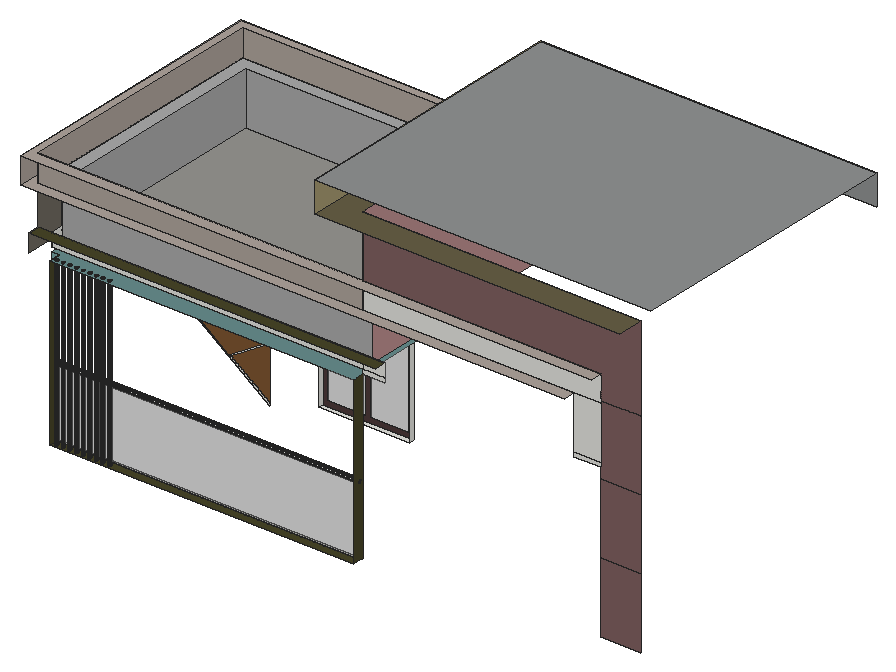
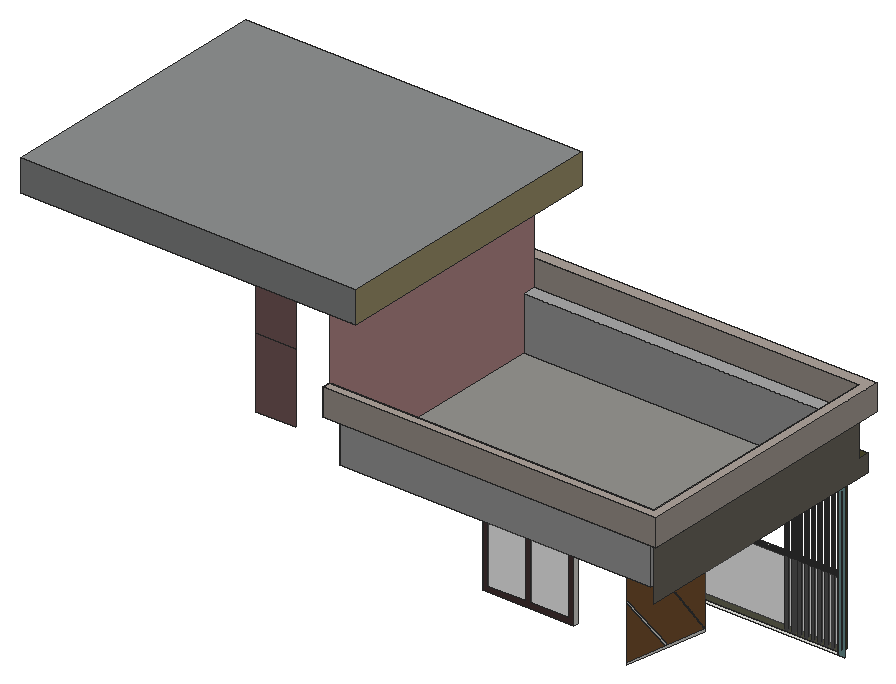
# SketchUp Ruby script. Lengths in inches.
U = 1.inch
M = Sketchup.active_model
def pt(a) = Geom::Point3d.new(a.map { |v| v * U })
def face(e, loops, mat)
  f = e.add_face(loops[0].map { |a| pt(a) })
  loops[1..].each { |l| e.add_face(l.map { |a| pt(a) }).erase! }
  f.material = f.back_material = mat if mat
  f
end
# faces: each face lists its corners as indices into pts; further lists are holes
def faces(e, pts, list, mat = nil) = list.each { |f| face(e, (f[0].is_a?(Array) ? f : [f]).map { |l| l.map { |i| pts[i] } }, mat) }
# xy, xz, yz: faces in a plane at the given z, y or x. An outline is a flat list of corners, or four numbers for a rectangle; further outlines are holes
def ring(l) = l.size == 4 ? [[l[0], l[1]], [l[2], l[1]], [l[2], l[3]], [l[0], l[3]]] : l.each_slice(2).to_a
def flat(e, list, mat, &to3) = list.each { |f| face(e, (f[0].is_a?(Array) ? f : [f]).map { |l| ring(l).map { |u, v| to3.(u, v) } }, mat) }
def xy(e, z, list, mat = nil) = flat(e, list, mat) { |x, y| [x, y, z] }
def xz(e, y, list, mat = nil) = flat(e, list, mat) { |x, z| [x, y, z] }
def yz(e, x, list, mat = nil) = flat(e, list, mat) { |y, z| [x, y, z] }
def lines(e, pts, list) = list.each { |a, b| e.add_line(pt(pts[a]), pt(pts[b])) }
# prism: a flat outline (further loops are holes) pulled along v
def prism(e, loops, v, mat = nil)
  f = face(e, loops, mat); d = Geom::Vector3d.new(v.map { |x| x * U })
  f.pushpull(f.normal.samedirection?(d) ? d.length : -d.length)
end
def box(e, o, s, mat = nil) = prism(e, [[o, [o[0] + s[0], o[1], o[2]], [o[0] + s[0], o[1] + s[1], o[2]], [o[0], o[1] + s[1], o[2]]]], [0, 0, s[2]], mat)
def at(x, y, z, deg = 0) = Geom::Transformation.translation(pt([x, y, z])) * Geom::Transformation.rotation(ORIGIN, Z_AXIS, deg.degrees)
def axes(o, x, y, z) = Geom::Transformation.new([*x, 0, *y, 0, *z, 0, *pt(o).to_a, 1])
def part(name) = M.definitions.add(name)
# library, detail: a bought-in or finely detailed component or shape, given as its bounding box
def library(name, o, s) = part(name).tap { |d| box(d.entities, o, s) }
def detail(e, o, s) = box(e.add_group.entities, o, s)
def put(e, d, t, mat = nil) = e.add_instance(d, t).tap { |i| i.material = mat if mat }
def group(e, t, mat = nil) = e.add_group.tap { |g| g.transformation = t; g.material = mat if mat }.entities
root = M.entities
M.materials.add("[0057_DarkKhaki]").color = [71, 69, 40]
M.materials.add("[0089_PaleTurquoise]").color = [103, 140, 140]
M.materials.add("[0089_PaleTurquoise]1").color = [120, 163, 163]
M.materials.add("[0119_RosyBrown]").color = [127, 96, 96]
M.materials.add("[0119_RosyBrown]1").color = [76, 58, 58]
M.materials.add("[0119_RosyBrown]2").color = [188, 143, 143]
M.materials.add("[0132_LightGray]1").color = [169, 169, 169]
M.materials.add("[Blacktop Old 02]").color = [143, 145, 145]
M.materials.add("[Cladding Stucco White]").color = [173, 163, 155]
M.materials.add("[Cladding Weathered]").color = [111, 105, 96]
M.materials.add("[Granite Light Gray]1").color = [149, 148, 144]
M.materials.add("[Translucent Glass Gray]").color = [130, 130, 130]
M.materials["[Translucent Glass Gray]"].alpha = 0.5
M.materials.add("[Translucent Glass Gray]1").color = [128, 128, 128]
M.materials["[Translucent Glass Gray]1"].alpha = 0.5
M.materials.add("[Wood Floor]").color = [124, 84, 49]
M.materials.add("[Wood Lumber ButtJoined]").color = [102, 94, 69]
M.materials.add("[Wood Lumber ButtJoined]3").color = [164, 152, 112]
xy(root,2010,[[306.11,174.36,305.08,174.5,304.11,174.9,303.29,175.53,302.65,176.36,302.25,177.32,302.11,178.36,302.25,179.4,302.65,180.36,303.29,181.1875,304.11,181.82,305.08,182.22,306.11,182.36,307.15,182.22,308.11,181.82,308.94,181.1875,309.58,180.36,309.98,179.4,310.11,178.36,309.98,177.32,309.58,176.36,308.94,175.53,308.11,174.9,307.15,174.5],[296.4,189.72,1122,198]])
xy(root,2010,[[[296.4,167,1122,189.72],[324.11,174.36,323.08,174.5,322.11,174.9,321.29,175.53,320.65,176.36,320.25,177.32,320.11,178.36,320.25,179.4,320.65,180.36,321.29,181.1875,322.11,181.82,323.08,182.22,324.11,182.36,325.15,182.22,326.11,181.82,326.94,181.1875,327.58,180.36,327.98,179.4,328.11,178.36,327.98,177.32,327.58,176.36,326.94,175.53,326.11,174.9,325.15,174.5],[342.11,174.36,341.08,174.5,340.11,174.9,339.29,175.53,338.65,176.36,338.25,177.32,338.11,178.36,338.25,179.4,338.65,180.36,339.29,181.1875,340.11,181.82,341.08,182.22,342.11,182.36,343.15,182.22,344.11,181.82,344.94,181.1875,345.58,180.36,345.98,179.4,346.11,178.36,345.98,177.32,345.58,176.36,344.94,175.53,344.11,174.9,343.15,174.5],[360.11,174.36,359.08,174.5,358.11,174.9,357.29,175.53,356.65,176.36,356.25,177.32,356.11,178.36,356.25,179.4,356.65,180.36,357.29,181.1875,358.11,181.82,359.08,182.22,360.11,182.36,361.15,182.22,362.11,181.82,362.94,181.1875,363.58,180.36,363.98,179.4,364.11,178.36,363.98,177.32,363.58,176.36,362.94,175.53,362.11,174.9,361.15,174.5],[378.11,174.36,377.08,174.5,376.11,174.9,375.29,175.53,374.65,176.36,374.25,177.32,374.11,178.36,374.25,179.4,374.65,180.36,375.29,181.1875,376.11,181.82,377.08,182.22,378.11,182.36,379.15,182.22,380.11,181.82,380.94,181.1875,381.58,180.36,381.98,179.4,382.11,178.36,381.98,177.32,381.58,176.36,380.94,175.53,380.11,174.9,379.15,174.5],[396.11,174.36,395.08,174.5,394.11,174.9,393.29,175.53,392.65,176.36,392.25,177.32,392.11,178.36,392.25,179.4,392.65,180.36,393.29,181.1875,394.11,181.82,395.08,182.22,396.11,182.36,397.15,182.22,398.11,181.82,398.94,181.1875,399.58,180.36,399.98,179.4,400.11,178.36,399.98,177.32,399.58,176.36,398.94,175.53,398.11,174.9,397.15,174.5],[414.11,174.36,413.08,174.5,412.11,174.9,411.29,175.53,410.65,176.36,410.25,177.32,410.11,178.36,410.25,179.4,410.65,180.36,411.29,181.1875,412.11,181.82,413.08,182.22,414.11,182.36,415.15,182.22,416.11,181.82,416.94,181.1875,417.58,180.36,417.98,179.4,418.11,178.36,417.98,177.32,417.58,176.36,416.94,175.53,416.11,174.9,415.15,174.5],[432.11,174.36,431.08,174.5,430.11,174.9,429.29,175.53,428.65,176.36,428.25,177.32,428.11,178.36,428.25,179.4,428.65,180.36,429.29,181.1875,430.11,181.82,431.08,182.22,432.11,182.36,433.15,182.22,434.11,181.82,434.94,181.1875,435.58,180.36,435.98,179.4,436.11,178.36,435.98,177.32,435.58,176.36,434.94,175.53,434.11,174.9,433.15,174.5],[450.11,174.36,449.08,174.5,448.11,174.9,447.29,175.53,446.65,176.36,446.25,177.32,446.11,178.36,446.25,179.4,446.65,180.36,447.29,181.1875,448.11,181.82,449.08,182.22,450.11,182.36,451.15,182.22,452.11,181.82,452.94,181.1875,453.58,180.36,453.98,179.4,454.11,178.36,453.98,177.32,453.58,176.36,452.94,175.53,452.11,174.9,451.15,174.5],[306.11,174.36,305.08,174.5,304.11,174.9,303.29,175.53,302.65,176.36,302.25,177.32,302.11,178.36,302.25,179.4,302.65,180.36,303.29,181.1875,304.11,181.82,305.08,182.22,306.11,182.36,307.15,182.22,308.11,181.82,308.94,181.1875,309.58,180.36,309.98,179.4,310.11,178.36,309.98,177.32,309.58,176.36,308.94,175.53,308.11,174.9,307.15,174.5]]],"[0057_DarkKhaki]")
xy(root,2088,[[726,546,973.25,558]])
xy(root,2374.11,[[373.89,546,586.11,552]])
xy(root,2388,[[726,546,973.25,558]])
xy(root,2460,[[411.39,218.73,408.29,219.14,405.39,220.34,402.91,222.25,401,224.73,399.8,227.625,399.39,230.73,399.8,233.84,401,236.73,402.91,239.22,405.39,241.125,408.29,242.32,411.39,242.73,414.5,242.32,417.39,241.125,419.88,239.22,421.79,236.73,422.99,233.84,423.39,230.73,422.99,227.625,421.79,224.73,419.88,222.25,417.39,220.34,414.5,219.14],[735.39,218.73,732.29,219.14,729.39,220.34,726.91,222.25,725,224.73,723.8,227.625,723.39,230.73,723.8,233.84,725,236.73,726.91,239.22,729.39,241.125,732.29,242.32,735.39,242.73,738.5,242.32,741.39,241.125,743.88,239.22,745.79,236.73,746.99,233.84,747.39,230.73,746.99,227.625,745.79,224.73,743.88,222.25,741.39,220.34,738.5,219.14],[1059.39,218.73,1056.29,219.14,1053.39,220.34,1050.91,222.25,1049,224.73,1047.8,227.625,1047.39,230.73,1047.8,233.84,1049,236.73,1050.91,239.22,1053.39,241.125,1056.29,242.32,1059.39,242.73,1062.5,242.32,1065.39,241.125,1067.88,239.22,1069.79,236.73,1070.99,233.84,1071.39,230.73,1070.99,227.625,1069.79,224.73,1067.88,222.25,1065.39,220.34,1062.5,219.14],[411.39,338.73,408.29,339.14,405.39,340.34,402.91,342.25,401,344.73,399.8,347.625,399.39,350.73,399.8,353.84,401,356.73,402.91,359.22,405.39,361.125,408.29,362.32,411.39,362.73,414.5,362.32,417.39,361.125,419.88,359.22,421.79,356.73,422.99,353.84,423.39,350.73,422.99,347.625,421.79,344.73,419.88,342.25,417.39,340.34,414.5,339.14],[735.39,338.73,732.29,339.14,729.39,340.34,726.91,342.25,725,344.73,723.8,347.625,723.39,350.73,723.8,353.84,725,356.73,726.91,359.22,729.39,361.125,732.29,362.32,735.39,362.73,738.5,362.32,741.39,361.125,743.88,359.22,745.79,356.73,746.99,353.84,747.39,350.73,746.99,347.625,745.79,344.73,743.88,342.25,741.39,340.34,738.5,339.14],
  [1059.39,338.73,1056.29,339.14,1053.39,340.34,1050.91,342.25,1049,344.73,1047.8,347.625,1047.39,350.73,1047.8,353.84,1049,356.73,1050.91,359.22,1053.39,361.125,1056.29,362.32,1059.39,362.73,1062.5,362.32,1065.39,361.125,1067.88,359.22,1069.79,356.73,1070.99,353.84,1071.39,350.73,1070.99,347.625,1069.79,344.73,1067.88,342.25,1065.39,340.34,1062.5,339.14]])
xy(root,2460,[[[296.4,167,296.4,198,276,198,276,546,1122,546,1122,167],[1059.39,218.73,1062.5,219.14,1065.39,220.34,1067.88,222.25,1069.79,224.73,1070.99,227.625,1071.39,230.73,1070.99,233.84,1069.79,236.73,1067.88,239.22,1065.39,241.125,1062.5,242.32,1059.39,242.73,1056.29,242.32,1053.39,241.125,1050.91,239.22,1049,236.73,1047.8,233.84,1047.39,230.73,1047.8,227.625,1049,224.73,1050.91,222.25,1053.39,220.34,1056.29,219.14],[411.39,218.73,414.5,219.14,417.39,220.34,419.88,222.25,421.79,224.73,422.99,227.625,423.39,230.73,422.99,233.84,421.79,236.73,419.88,239.22,417.39,241.125,414.5,242.32,411.39,242.73,408.29,242.32,405.39,241.125,402.91,239.22,401,236.73,399.8,233.84,399.39,230.73,399.8,227.625,401,224.73,402.91,222.25,405.39,220.34,408.29,219.14],[411.39,338.73,414.5,339.14,417.39,340.34,419.88,342.25,421.79,344.73,422.99,347.625,423.39,350.73,422.99,353.84,421.79,356.73,419.88,359.22,417.39,361.125,414.5,362.32,411.39,362.73,408.29,362.32,405.39,361.125,402.91,359.22,401,356.73,399.8,353.84,399.39,350.73,399.8,347.625,401,344.73,402.91,342.25,405.39,340.34,408.29,339.14],[735.39,338.73,738.5,339.14,741.39,340.34,743.88,342.25,745.79,344.73,746.99,347.625,747.39,350.73,746.99,353.84,745.79,356.73,743.88,359.22,741.39,361.125,738.5,362.32,735.39,362.73,732.29,362.32,729.39,361.125,726.91,359.22,725,356.73,723.8,353.84,723.39,350.73,723.8,347.625,725,344.73,726.91,342.25,729.39,340.34,732.29,339.14],[1059.39,338.73,1062.5,339.14,1065.39,340.34,1067.88,342.25,1069.79,344.73,1070.99,347.625,1071.39,350.73,1070.99,353.84,1069.79,356.73,1067.88,359.22,1065.39,361.125,1062.5,362.32,1059.39,362.73,1056.29,362.32,1053.39,361.125,1050.91,359.22,1049,356.73,1047.8,353.84,1047.39,350.73,1047.8,347.625,1049,344.73,1050.91,342.25,1053.39,340.34,1056.29,339.14],[735.39,218.73,738.5,219.14,741.39,220.34,743.88,222.25,745.79,224.73,746.99,227.625,747.39,230.73,746.99,233.84,745.79,236.73,743.88,239.22,741.39,241.125,738.5,242.32,735.39,242.73,732.29,242.32,729.39,241.125,726.91,239.22,725,236.73,723.8,233.84,723.39,230.73,723.8,227.625,725,224.73,726.91,222.25,729.39,220.34,732.29,219.14],[306.11,174.36,307.15,174.5,308.11,174.9,308.94,175.53,309.58,176.36,309.98,177.32,310.11,178.36,309.98,179.4,309.58,180.36,308.94,181.1875,308.11,181.82,307.15,182.22,306.11,182.36,305.08,182.22,304.11,181.82,303.29,181.1875,302.65,180.36,302.25,179.4,302.11,178.36,302.25,177.32,302.65,176.36,303.29,175.53,304.11,174.9,305.08,174.5],[324.11,174.36,325.15,174.5,326.11,174.9,326.94,175.53,327.58,176.36,327.98,177.32,328.11,178.36,327.98,179.4,327.58,180.36,326.94,181.1875,326.11,181.82,325.15,182.22,324.11,182.36,323.08,182.22,322.11,181.82,321.29,181.1875,320.65,180.36,320.25,179.4,320.11,178.36,320.25,177.32,320.65,176.36,321.29,175.53,322.11,174.9,323.08,174.5],[342.11,174.36,343.15,174.5,344.11,174.9,344.94,175.53,345.58,176.36,345.98,177.32,346.11,178.36,345.98,179.4,345.58,180.36,344.94,181.1875,344.11,181.82,343.15,182.22,342.11,182.36,341.08,182.22,340.11,181.82,339.29,181.1875,338.65,180.36,338.25,179.4,338.11,178.36,338.25,177.32,338.65,176.36,339.29,175.53,340.11,174.9,341.08,174.5],[360.11,174.36,361.15,174.5,362.11,174.9,362.94,175.53,363.58,176.36,363.98,177.32,364.11,178.36,363.98,179.4,363.58,180.36,362.94,181.1875,362.11,181.82,361.15,182.22,360.11,182.36,359.08,182.22,358.11,181.82,357.29,181.1875,356.65,180.36,356.25,179.4,356.11,178.36,356.25,177.32,356.65,176.36,357.29,175.53,358.11,174.9,359.08,174.5],[378.11,174.36,379.15,174.5,380.11,174.9,380.94,175.53,381.58,176.36,381.98,177.32,382.11,178.36,381.98,179.4,381.58,180.36,380.94,181.1875,380.11,181.82,379.15,182.22,378.11,182.36,377.08,182.22,376.11,181.82,375.29,181.1875,374.65,180.36,374.25,179.4,374.11,178.36,374.25,177.32,374.65,176.36,375.29,175.53,376.11,174.9,377.08,174.5],[396.11,174.36,397.15,174.5,398.11,174.9,398.94,175.53,399.58,176.36,399.98,177.32,400.11,178.36,399.98,179.4,399.58,180.36,398.94,181.1875,398.11,181.82,397.15,182.22,396.11,182.36,395.08,182.22,394.11,181.82,393.29,181.1875,392.65,180.36,392.25,179.4,392.11,178.36,392.25,177.32,392.65,176.36,393.29,175.53,394.11,174.9,395.08,174.5],[414.11,174.36,415.15,174.5,416.11,174.9,416.94,175.53,417.58,176.36,417.98,177.32,418.11,178.36,417.98,179.4,417.58,180.36,416.94,181.1875,416.11,181.82,415.15,182.22,414.11,182.36,413.08,182.22,412.11,181.82,411.29,181.1875,410.65,180.36,410.25,179.4,410.11,178.36,410.25,177.32,410.65,176.36,411.29,175.53,412.11,174.9,413.08,174.5],[432.11,174.36,433.15,174.5,434.11,174.9,434.94,175.53,435.58,176.36,435.98,177.32,436.11,178.36,435.98,179.4,435.58,180.36,434.94,181.1875,434.11,181.82,433.15,182.22,432.11,182.36,431.08,182.22,430.11,181.82,429.29,181.1875,428.65,180.36,428.25,179.4,428.11,178.36,428.25,177.32,428.65,176.36,429.29,175.53,430.11,174.9,431.08,174.5],[450.11,174.36,451.15,174.5,452.11,174.9,452.94,175.53,453.58,176.36,453.98,177.32,454.11,178.36,453.98,179.4,453.58,180.36,452.94,181.1875,452.11,181.82,451.15,182.22,450.11,182.36,449.08,182.22,448.11,181.82,447.29,181.1875,446.65,180.36,446.25,179.4,446.11,178.36,446.25,177.32,446.65,176.36,447.29,175.53,448.11,174.9,449.08,174.5]]],"[0089_PaleTurquoise]")
xy(root,2472,[[276.25,198,1122,234]])
xy(root,2472,[[276.25,234,1122,858]],"[Granite Light Gray]1")
xy(root,2508,[[240,167,1182,198]],"[0057_DarkKhaki]")
xy(root,2616,[[240,198,1122,198,1122,234,276.25,234,276.25,858,1122,858,1122,894,240,894]],"[0132_LightGray]1")
xy(root,2616,[[216,167,216,918,1122,918,1122,894,240,894,240,198,1698,198,1698,167]],"[Cladding Stucco White]")
xy(root,2688,[[216,167,1770,167,1770,198,240,198,240,894,1122,894,1122,918,216,918]],"[Cladding Stucco White]")
xy(root,2856,[[1050,126,1050,894,1122,894,1122,198,1879.2,198,1879.2,126]],"[Wood Lumber ButtJoined]")
xy(root,2940,[[1050,126,1963.2,894]],"[Blacktop Old 02]")
xz(root,189.72,[[296.4,2010,1122,2196]],"[Translucent Glass Gray]")
xz(root,198,[[1122,2460,1182,2472],[1698,2460,1770,2472],[276.25,2472,1122,2508],[1122,2472,1182,2508],[1698,2472,1770,2616],
  [1122,2616,1770,2688]])
xz(root,198,[[276,2010,296.4,2460]],"[0089_PaleTurquoise]1")
xz(root,198,[[1770,2046.875,1879.2,2238.875],[1770,2238.875,1879.2,2430.875],[1770,2430.875,1879.2,2622.875],[1770,2622.875,1879.2,2622.875,1879.2,2856,1122,2856,1122,2688,1770,2688]],"[0119_RosyBrown]")
xz(root,198,[[240,2616,1122,2688]],"[Cladding Stucco White]")
xz(root,234,[[276.25,2472,1122,2616]],"[0132_LightGray]1")
xz(root,552,[[586.11,2039.4,586.11,2044.94,480,2122.72,476.37,2125.38,373.89,2200.5,373.89,2194.56],[480,2122.72,586.11,2189.8,586.11,2194.15,476.37,2125.38],[373.89,2200.5,586.11,2357.37,586.11,2361.5,503.08,2300.04,498.99,2297.01,373.89,2204.42],[498.99,2297.01,503.08,2300.04,380.08,2374.11,373.89,2374.11]])
xz(root,552,[[586.11,2044.94,586.11,2189.8,480,2122.72],[476.37,2125.38,586.11,2194.15,586.11,2357.37,373.89,2200.5],[373.89,2204.42,498.99,2297.01,373.89,2374.11],[503.08,2300.04,586.11,2361.5,586.11,2374.11,380.08,2374.11]],"[Wood Floor]")
xz(root,558,[[[726,2088,973.25,2388],[855.625,2101.89,959.36,2374.11],[739.89,2101.89,843.625,2374.11]]],"[0119_RosyBrown]1")
xz(root,558,[[739.89,2101.89,843.625,2374.11],[855.625,2101.89,959.36,2374.11]],"[Translucent Glass Gray]1")
xz(root,858,[[276.25,2472,1122,2616]],"[0132_LightGray]1")
xz(root,894,[[1050,2856,1963.2,2940]],"[Blacktop Old 02]")
xz(root,894,[[240,2616,1122,2688]],"[Cladding Stucco White]")
xz(root,918,[[216,2616,1122,2688]],"[Cladding Stucco White]")
yz(root,216,[[167,2616,918,2688]],"[Cladding Stucco White]")
yz(root,240,[[198,2616,894,2688]],"[Cladding Stucco White]")
yz(root,240,[[167,2460,167,2508,198,2508,198,2616,894,2616,894,2460]],"[Cladding Weathered]")
yz(root,276.25,[[198,2472,234,2508]])
yz(root,276.25,[[234,2472,858,2616]],"[0132_LightGray]1")
yz(root,296.4,[[189.72,2196,188.17,2196.2,186.72,2196.8,185.48,2197.76,184.52,2199,183.92,2200.45,183.72,2202,183.92,2203.55,184.52,2205,185.48,2206.24,186.72,2207.2,188.17,2207.8,189.72,2208,191.27,2207.8,192.72,2207.2,193.96,2206.24,194.92,2205,195.52,2203.55,195.72,2202,195.52,2200.45,194.92,2199,193.96,2197.76,192.72,2196.8,191.27,2196.2]])
yz(root,296.4,[[[167,2010,198,2460],[189.72,2196,188.17,2196.2,186.72,2196.8,185.48,2197.76,184.52,2199,183.92,2200.45,183.72,2202,183.92,2203.55,184.52,2205,185.48,2206.24,186.72,2207.2,188.17,2207.8,189.72,2208,191.27,2207.8,192.72,2207.2,193.96,2206.24,194.92,2205,195.52,2203.55,195.72,2202,195.52,2200.45,194.92,2199,193.96,2197.76,192.72,2196.8,191.27,2196.2]]],"[0057_DarkKhaki]")
yz(root,726,[[546,2088,558,2388]])
yz(root,973.25,[[546,2088,558,2388]])
yz(root,1050,[[126,2856,894,2940]],"[Wood Lumber ButtJoined]3")
yz(root,1122,[[894,2616,918,2688]])
yz(root,1122,[[167,2010,167,2460,198,2460,198,2010,189.72,2010,189.72,2196,191.27,2196.2,192.72,2196.8,193.96,2197.76,194.92,2199,195.52,2200.45,195.72,2202,195.52,2203.55,194.92,2205,193.96,2206.24,192.72,2207.2,191.27,2207.8,189.72,2208,188.17,2207.8,186.72,2207.2,185.48,2206.24,184.52,2205,183.92,2203.55,183.72,2202,183.92,2200.45,184.52,2199,185.48,2197.76,186.72,2196.8,188.17,2196.2,189.72,2196,189.72,2010]],"[0057_DarkKhaki]")
yz(root,1122,[[234,2472,234,2616,198,2616,198,2856,894,2856,894,2616,858,2616,858,2472]],"[0119_RosyBrown]2")
p = [[305.08,174.5,2010],[306.11,174.36,2010],[306.11,174.36,2460],[305.08,174.5,2460],[307.15,174.5,2010],[307.15,174.5,2460],
  [323.08,174.5,2010],[324.11,174.36,2010],[324.11,174.36,2460],[323.08,174.5,2460],[325.15,174.5,2010],[325.15,174.5,2460],
  [341.08,174.5,2010],[342.11,174.36,2010],[342.11,174.36,2460],[341.08,174.5,2460],[343.15,174.5,2010],[343.15,174.5,2460],
  [359.08,174.5,2010],[360.11,174.36,2010],[360.11,174.36,2460],[359.08,174.5,2460],[361.15,174.5,2010],[361.15,174.5,2460],
  [377.08,174.5,2010],[378.11,174.36,2010],[378.11,174.36,2460],[377.08,174.5,2460],[379.15,174.5,2010],[379.15,174.5,2460],
  [395.08,174.5,2010],[396.11,174.36,2010],[396.11,174.36,2460],[395.08,174.5,2460],[397.15,174.5,2010],[397.15,174.5,2460],
  [413.08,174.5,2010],[414.11,174.36,2010],[414.11,174.36,2460],[413.08,174.5,2460],[415.15,174.5,2010],[415.15,174.5,2460],
  [431.08,174.5,2010],[432.11,174.36,2010],[432.11,174.36,2460],[431.08,174.5,2460],[433.15,174.5,2010],[433.15,174.5,2460],
  [449.08,174.5,2010],[450.11,174.36,2010],[450.11,174.36,2460],[449.08,174.5,2460],[451.15,174.5,2010],[451.15,174.5,2460],
  [304.11,174.9,2010],[304.11,174.9,2460],[308.11,174.9,2010],[308.11,174.9,2460],[322.11,174.9,2010],[322.11,174.9,2460],
  [326.11,174.9,2010],[326.11,174.9,2460],[340.11,174.9,2010],[340.11,174.9,2460],[344.11,174.9,2010],[344.11,174.9,2460],
  [358.11,174.9,2010],[358.11,174.9,2460],[362.11,174.9,2010],[362.11,174.9,2460],[376.11,174.9,2010],[376.11,174.9,2460],
  [380.11,174.9,2010],[380.11,174.9,2460],[394.11,174.9,2010],[394.11,174.9,2460],[398.11,174.9,2010],[398.11,174.9,2460],
  [412.11,174.9,2010],[412.11,174.9,2460],[416.11,174.9,2010],[416.11,174.9,2460],[430.11,174.9,2010],[430.11,174.9,2460],
  [434.11,174.9,2010],[434.11,174.9,2460],[448.11,174.9,2010],[448.11,174.9,2460],[452.11,174.9,2010],[452.11,174.9,2460],
  [303.29,175.53,2010],[303.29,175.53,2460],[308.94,175.53,2010],[308.94,175.53,2460],[321.29,175.53,2010],[321.29,175.53,2460],
  [326.94,175.53,2010],[326.94,175.53,2460],[339.29,175.53,2010],[339.29,175.53,2460],[344.94,175.53,2010],[344.94,175.53,2460],
  [357.29,175.53,2010],[357.29,175.53,2460],[362.94,175.53,2010],[362.94,175.53,2460],[375.29,175.53,2010],[375.29,175.53,2460],
  [380.94,175.53,2010],[380.94,175.53,2460],[393.29,175.53,2010],[393.29,175.53,2460],[398.94,175.53,2010],[398.94,175.53,2460],
  [411.29,175.53,2010],[411.29,175.53,2460],[416.94,175.53,2010],[416.94,175.53,2460],[429.29,175.53,2010],[429.29,175.53,2460],
  [434.94,175.53,2010],[434.94,175.53,2460],[447.29,175.53,2010],[447.29,175.53,2460],[452.94,175.53,2010],[452.94,175.53,2460],
  [302.65,176.36,2010],[302.65,176.36,2460],[309.58,176.36,2010],[309.58,176.36,2460],[320.65,176.36,2010],[320.65,176.36,2460],
  [327.58,176.36,2010],[327.58,176.36,2460],[338.65,176.36,2010],[338.65,176.36,2460],[345.58,176.36,2010],[345.58,176.36,2460],
  [356.65,176.36,2010],[356.65,176.36,2460],[363.58,176.36,2010],[363.58,176.36,2460],[374.65,176.36,2010],[374.65,176.36,2460],
  [381.58,176.36,2010],[381.58,176.36,2460],[392.65,176.36,2010],[392.65,176.36,2460],[399.58,176.36,2010],[399.58,176.36,2460],
  [410.65,176.36,2010],[410.65,176.36,2460],[417.58,176.36,2010],[417.58,176.36,2460],[428.65,176.36,2010],[428.65,176.36,2460],
  [435.58,176.36,2010],[435.58,176.36,2460],[446.65,176.36,2010],[446.65,176.36,2460],[453.58,176.36,2010],[453.58,176.36,2460],
  [302.25,177.32,2010],[302.25,177.32,2460],[309.98,177.32,2010],[309.98,177.32,2460],[320.25,177.32,2010],[320.25,177.32,2460],
  [327.98,177.32,2010],[327.98,177.32,2460],[338.25,177.32,2010],[338.25,177.32,2460],[345.98,177.32,2010],[345.98,177.32,2460],
  [356.25,177.32,2010],[356.25,177.32,2460],[363.98,177.32,2010],[363.98,177.32,2460],[374.25,177.32,2010],[374.25,177.32,2460],
  [381.98,177.32,2010],[381.98,177.32,2460],[392.25,177.32,2010],[392.25,177.32,2460],[399.98,177.32,2010],[399.98,177.32,2460],
  [410.25,177.32,2010],[410.25,177.32,2460],[417.98,177.32,2010],[417.98,177.32,2460],[428.25,177.32,2010],[428.25,177.32,2460],
  [435.98,177.32,2010],[435.98,177.32,2460],[446.25,177.32,2010],[446.25,177.32,2460],[453.98,177.32,2010],[453.98,177.32,2460],
  [302.11,178.36,2010],[302.11,178.36,2460],[310.11,178.36,2010],[310.11,178.36,2460],[320.11,178.36,2010],[320.11,178.36,2460],
  [328.11,178.36,2010],[328.11,178.36,2460],[338.11,178.36,2010],[338.11,178.36,2460],[346.11,178.36,2010],[346.11,178.36,2460],
  [356.11,178.36,2010],[356.11,178.36,2460],[364.11,178.36,2010],[364.11,178.36,2460],[374.11,178.36,2010],[374.11,178.36,2460],
  [382.11,178.36,2010],[382.11,178.36,2460],[392.11,178.36,2010],[392.11,178.36,2460],[400.11,178.36,2010],[400.11,178.36,2460],
  [410.11,178.36,2010],[410.11,178.36,2460],[418.11,178.36,2010],[418.11,178.36,2460],[428.11,178.36,2010],[428.11,178.36,2460],
  [436.11,178.36,2010],[436.11,178.36,2460],[446.11,178.36,2010],[446.11,178.36,2460],[454.11,178.36,2010],[454.11,178.36,2460],
  [302.25,179.4,2010],[302.25,179.4,2460],[309.98,179.4,2010],[309.98,179.4,2460],[320.25,179.4,2010],[320.25,179.4,2460],
  [327.98,179.4,2010],[327.98,179.4,2460],[338.25,179.4,2010],[338.25,179.4,2460],[345.98,179.4,2010],[345.98,179.4,2460],
  [356.25,179.4,2010],[356.25,179.4,2460],[363.98,179.4,2010],[363.98,179.4,2460],[374.25,179.4,2010],[374.25,179.4,2460],
  [381.98,179.4,2010],[381.98,179.4,2460],[392.25,179.4,2010],[392.25,179.4,2460],[399.98,179.4,2010],[399.98,179.4,2460],
  [410.25,179.4,2010],[410.25,179.4,2460],[417.98,179.4,2010],[417.98,179.4,2460],[428.25,179.4,2010],[428.25,179.4,2460],
  [435.98,179.4,2010],[435.98,179.4,2460],[446.25,179.4,2010],[446.25,179.4,2460],[453.98,179.4,2010],[453.98,179.4,2460],
  [302.65,180.36,2010],[302.65,180.36,2460],[309.58,180.36,2010],[309.58,180.36,2460],[320.65,180.36,2010],[320.65,180.36,2460],
  [327.58,180.36,2010],[327.58,180.36,2460],[338.65,180.36,2010],[338.65,180.36,2460],[345.58,180.36,2010],[345.58,180.36,2460],
  [356.65,180.36,2010],[356.65,180.36,2460],[363.58,180.36,2010],[363.58,180.36,2460],[374.65,180.36,2010],[374.65,180.36,2460],
  [381.58,180.36,2010],[381.58,180.36,2460],[392.65,180.36,2010],[392.65,180.36,2460],[399.58,180.36,2010],[399.58,180.36,2460],
  [410.65,180.36,2010],[410.65,180.36,2460],[417.58,180.36,2010],[417.58,180.36,2460],[428.65,180.36,2010],[428.65,180.36,2460],
  [435.58,180.36,2010],[435.58,180.36,2460],[446.65,180.36,2010],[446.65,180.36,2460],[453.58,180.36,2010],[453.58,180.36,2460],
  [303.29,181.1875,2010],[303.29,181.1875,2460],[308.94,181.1875,2010],[308.94,181.1875,2460],[321.29,181.1875,2010],[321.29,181.1875,2460],
  [326.94,181.1875,2010],[326.94,181.1875,2460],[339.29,181.1875,2010],[339.29,181.1875,2460],[344.94,181.1875,2010],[344.94,181.1875,2460],
  [357.29,181.1875,2010],[357.29,181.1875,2460],[362.94,181.1875,2010],[362.94,181.1875,2460],[375.29,181.1875,2010],[375.29,181.1875,2460],
  [380.94,181.1875,2010],[380.94,181.1875,2460],[393.29,181.1875,2010],[393.29,181.1875,2460],[398.94,181.1875,2010],[398.94,181.1875,2460],
  [411.29,181.1875,2010],[411.29,181.1875,2460],[416.94,181.1875,2010],[416.94,181.1875,2460],[429.29,181.1875,2010],[429.29,181.1875,2460],
  [434.94,181.1875,2010],[434.94,181.1875,2460],[447.29,181.1875,2010],[447.29,181.1875,2460],[452.94,181.1875,2010],[452.94,181.1875,2460],
  [304.11,181.82,2010],[304.11,181.82,2460],[308.11,181.82,2010],[308.11,181.82,2460],[322.11,181.82,2010],[322.11,181.82,2460],
  [326.11,181.82,2010],[326.11,181.82,2460],[340.11,181.82,2010],[340.11,181.82,2460],[344.11,181.82,2010],[344.11,181.82,2460],
  [358.11,181.82,2010],[358.11,181.82,2460],[362.11,181.82,2010],[362.11,181.82,2460],[376.11,181.82,2010],[376.11,181.82,2460],
  [380.11,181.82,2010],[380.11,181.82,2460],[394.11,181.82,2010],[394.11,181.82,2460],[398.11,181.82,2010],[398.11,181.82,2460],
  [412.11,181.82,2010],[412.11,181.82,2460],[416.11,181.82,2010],[416.11,181.82,2460],[430.11,181.82,2010],[430.11,181.82,2460],
  [434.11,181.82,2010],[434.11,181.82,2460],[448.11,181.82,2010],[448.11,181.82,2460],[452.11,181.82,2010],[452.11,181.82,2460],
  [305.08,182.22,2010],[305.08,182.22,2460],[307.15,182.22,2010],[307.15,182.22,2460],[323.08,182.22,2010],[323.08,182.22,2460],
  [325.15,182.22,2010],[325.15,182.22,2460],[341.08,182.22,2010],[341.08,182.22,2460],[343.15,182.22,2010],[343.15,182.22,2460],
  [359.08,182.22,2010],[359.08,182.22,2460],[361.15,182.22,2010],[361.15,182.22,2460],[377.08,182.22,2010],[377.08,182.22,2460],
  [379.15,182.22,2010],[379.15,182.22,2460],[395.08,182.22,2010],[395.08,182.22,2460],[397.15,182.22,2010],[397.15,182.22,2460],
  [413.08,182.22,2010],[413.08,182.22,2460],[415.15,182.22,2010],[415.15,182.22,2460],[431.08,182.22,2010],[431.08,182.22,2460],
  [433.15,182.22,2010],[433.15,182.22,2460],[449.08,182.22,2010],[449.08,182.22,2460],[451.15,182.22,2010],[451.15,182.22,2460],
  [306.11,182.36,2010],[306.11,182.36,2460],[324.11,182.36,2010],[324.11,182.36,2460],[342.11,182.36,2010],[342.11,182.36,2460],
  [360.11,182.36,2010],[360.11,182.36,2460],[378.11,182.36,2010],[378.11,182.36,2460],[396.11,182.36,2010],[396.11,182.36,2460],
  [414.11,182.36,2010],[414.11,182.36,2460],[432.11,182.36,2010],[432.11,182.36,2460],[450.11,182.36,2010],[450.11,182.36,2460],
  [296.4,188.17,2196.2],[296.4,189.72,2196],[1122,189.72,2196],[1122,188.17,2196.2],[296.4,191.27,2196.2],[1122,191.27,2196.2],
  [296.4,186.72,2196.8],[1122,186.72,2196.8],[296.4,192.72,2196.8],[1122,192.72,2196.8],[296.4,185.48,2197.76],[1122,185.48,2197.76],
  [296.4,193.96,2197.76],[1122,193.96,2197.76],[296.4,184.52,2199],[1122,184.52,2199],[296.4,194.92,2199],[1122,194.92,2199],
  [296.4,183.92,2200.45],[1122,183.92,2200.45],[296.4,195.52,2200.45],[1122,195.52,2200.45],[296.4,183.72,2202],[1122,183.72,2202],
  [296.4,195.72,2202],[1122,195.72,2202],[296.4,183.92,2203.55],[1122,183.92,2203.55],[296.4,195.52,2203.55],[1122,195.52,2203.55],
  [296.4,184.52,2205],[1122,184.52,2205],[296.4,194.92,2205],[1122,194.92,2205],[296.4,185.48,2206.24],[1122,185.48,2206.24],
  [296.4,193.96,2206.24],[1122,193.96,2206.24],[296.4,186.72,2207.2],[1122,186.72,2207.2],[296.4,192.72,2207.2],[1122,192.72,2207.2],
  [296.4,188.17,2207.8],[1122,188.17,2207.8],[296.4,191.27,2207.8],[1122,191.27,2207.8],[296.4,189.72,2208],[1122,189.72,2208],
  [1122,189.72,2202],[296.4,189.72,2202]]
faces(root,p,[[0,1,2,3],[1,4,5,2],[6,7,8,9],[7,10,11,8],[12,13,14,15],[13,16,17,14],[18,19,20,21],[19,22,23,20],
  [24,25,26,27],[25,28,29,26],[30,31,32,33],[31,34,35,32],[36,37,38,39],[37,40,41,38],[42,43,44,45],[43,46,47,44],
  [48,49,50,51],[49,52,53,50],[54,0,3,55],[4,56,57,5],[58,6,9,59],[10,60,61,11],[62,12,15,63],[16,64,65,17],
  [66,18,21,67],[22,68,69,23],[70,24,27,71],[28,72,73,29],[74,30,33,75],[34,76,77,35],[78,36,39,79],[40,80,81,41],
  [82,42,45,83],[46,84,85,47],[86,48,51,87],[52,88,89,53],[90,54,55,91],[56,92,93,57],[94,58,59,95],[60,96,97,61],
  [98,62,63,99],[64,100,101,65],[102,66,67,103],[68,104,105,69],[106,70,71,107],[72,108,109,73],[110,74,75,111],[76,112,113,77],
  [114,78,79,115],[80,116,117,81],[118,82,83,119],[84,120,121,85],[122,86,87,123],[88,124,125,89],[126,90,91,127],[92,128,129,93],
  [130,94,95,131],[96,132,133,97],[134,98,99,135],[100,136,137,101],[138,102,103,139],[104,140,141,105],[142,106,107,143],[108,144,145,109],
  [146,110,111,147],[112,148,149,113],[150,114,115,151],[116,152,153,117],[154,118,119,155],[120,156,157,121],[158,122,123,159],[124,160,161,125],
  [162,126,127,163],[128,164,165,129],[166,130,131,167],[132,168,169,133],[170,134,135,171],[136,172,173,137],[174,138,139,175],[140,176,177,141],
  [178,142,143,179],[144,180,181,145],[182,146,147,183],[148,184,185,149],[186,150,151,187],[152,188,189,153],[190,154,155,191],[156,192,193,157],
  [194,158,159,195],[160,196,197,161],[198,162,163,199],[164,200,201,165],[202,166,167,203],[168,204,205,169],[206,170,171,207],[172,208,209,173],
  [210,174,175,211],[176,212,213,177],[214,178,179,215],[180,216,217,181],[218,182,183,219],[184,220,221,185],[222,186,187,223],[188,224,225,189],
  [226,190,191,227],[192,228,229,193],[230,194,195,231],[196,232,233,197],[234,198,199,235],[200,236,237,201],[238,202,203,239],[204,240,241,205],
  [242,206,207,243],[208,244,245,209],[246,210,211,247],[212,248,249,213],[250,214,215,251],[216,252,253,217],[254,218,219,255],[220,256,257,221],
  [258,222,223,259],[224,260,261,225],[262,226,227,263],[228,264,265,229],[266,230,231,267],[232,268,269,233],[270,234,235,271],[236,272,273,237],
  [274,238,239,275],[240,276,277,241],[278,242,243,279],[244,280,281,245],[282,246,247,283],[248,284,285,249],[286,250,251,287],[252,288,289,253],
  [290,254,255,291],[256,292,293,257],[294,258,259,295],[260,296,297,261],[298,262,263,299],[264,300,301,265],[302,266,267,303],[268,304,305,269],
  [306,270,271,307],[272,308,309,273],[310,274,275,311],[276,312,313,277],[314,278,279,315],[280,316,317,281],[318,282,283,319],[284,320,321,285],
  [322,286,287,323],[288,324,325,289],[326,290,291,327],[292,328,329,293],[330,294,295,331],[296,332,333,297],[334,298,299,335],[300,336,337,301],
  [338,302,303,339],[304,340,341,305],[342,306,307,343],[308,344,345,309],[346,310,311,347],[312,348,349,313],[350,314,315,351],[316,352,353,317],
  [354,318,319,355],[320,356,357,321],[358,322,323,359],[324,360,361,325],[362,326,327,363],[328,364,365,329],[366,330,331,367],[332,368,369,333],
  [370,334,335,371],[336,372,373,337],[374,338,339,375],[340,376,377,341],[378,342,343,379],[344,380,381,345],[382,346,347,383],[348,384,385,349],
  [386,350,351,387],[352,388,389,353],[390,354,355,391],[356,392,393,357],[394,358,359,395],[360,396,397,361],[398,362,363,399],[364,400,401,365],
  [402,366,367,403],[368,404,405,369],[406,370,371,407],[372,408,409,373],[410,374,375,411],[376,412,413,377],[414,378,379,415],[380,414,415,381],
  [416,382,383,417],[384,416,417,385],[418,386,387,419],[388,418,419,389],[420,390,391,421],[392,420,421,393],[422,394,395,423],[396,422,423,397],
  [424,398,399,425],[400,424,425,401],[426,402,403,427],[404,426,427,405],[428,406,407,429],[408,428,429,409],[430,410,411,431],[412,430,431,413]],"[0119_RosyBrown]")
faces(root,p,[[432,433,434,435],[433,436,437,434],[438,432,435,439],[436,440,441,437],[442,438,439,443],[440,444,445,441],[446,442,443,447],[444,448,449,445],
  [450,446,447,451],[448,452,453,449],[454,450,451,455],[452,456,457,453],[458,454,455,459],[456,460,461,457],[462,458,459,463],[460,464,465,461],
  [466,462,463,467],[464,468,469,465],[470,466,467,471],[468,472,473,469],[474,470,471,475],[472,476,477,473],[478,474,475,479],[476,478,479,477]])
lines(root,p,[[480,481],[434,480]])
